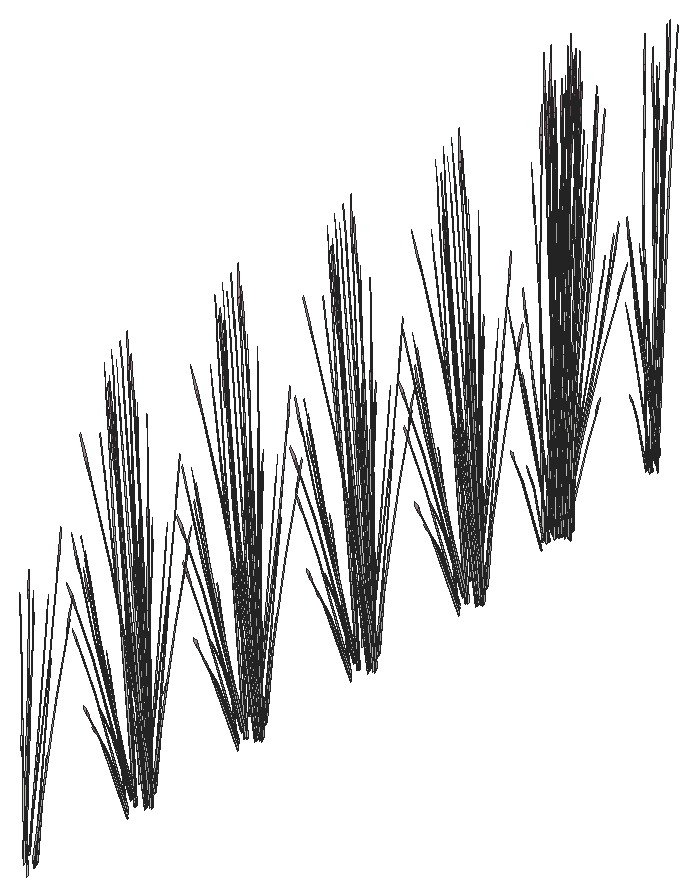
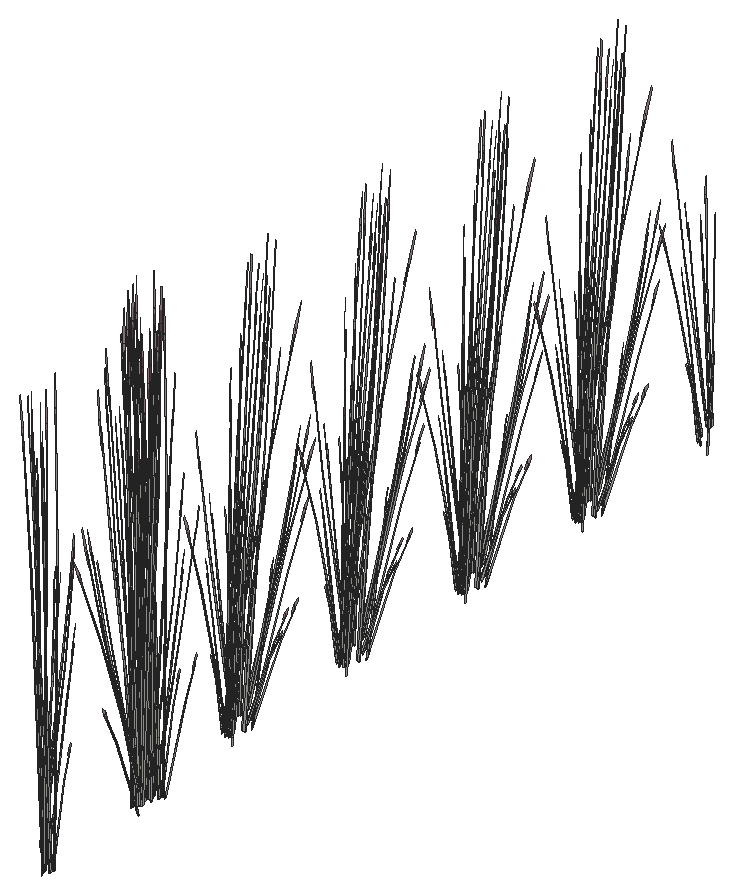
# SketchUp Ruby script. Lengths in inches.
U = 1.inch
M = Sketchup.active_model
def pt(a) = Geom::Point3d.new(a.map { |v| v * U })
def face(e, loops, mat)
  f = e.add_face(loops[0].map { |a| pt(a) })
  loops[1..].each { |l| e.add_face(l.map { |a| pt(a) }).erase! }
  f.material = f.back_material = mat if mat
  f
end
# faces: each face lists its corners as indices into pts; further lists are holes
def faces(e, pts, list, mat = nil) = list.each { |f| face(e, (f[0].is_a?(Array) ? f : [f]).map { |l| l.map { |i| pts[i] } }, mat) }
# xy, xz, yz: faces in a plane at the given z, y or x. An outline is a flat list of corners, or four numbers for a rectangle; further outlines are holes
def ring(l) = l.size == 4 ? [[l[0], l[1]], [l[2], l[1]], [l[2], l[3]], [l[0], l[3]]] : l.each_slice(2).to_a
def flat(e, list, mat, &to3) = list.each { |f| face(e, (f[0].is_a?(Array) ? f : [f]).map { |l| ring(l).map { |u, v| to3.(u, v) } }, mat) }
def xy(e, z, list, mat = nil) = flat(e, list, mat) { |x, y| [x, y, z] }
def xz(e, y, list, mat = nil) = flat(e, list, mat) { |x, z| [x, y, z] }
def yz(e, x, list, mat = nil) = flat(e, list, mat) { |y, z| [x, y, z] }
def lines(e, pts, list) = list.each { |a, b| e.add_line(pt(pts[a]), pt(pts[b])) }
# prism: a flat outline (further loops are holes) pulled along v
def prism(e, loops, v, mat = nil)
  f = face(e, loops, mat); d = Geom::Vector3d.new(v.map { |x| x * U })
  f.pushpull(f.normal.samedirection?(d) ? d.length : -d.length)
end
def box(e, o, s, mat = nil) = prism(e, [[o, [o[0] + s[0], o[1], o[2]], [o[0] + s[0], o[1] + s[1], o[2]], [o[0], o[1] + s[1], o[2]]]], [0, 0, s[2]], mat)
def at(x, y, z, deg = 0) = Geom::Transformation.translation(pt([x, y, z])) * Geom::Transformation.rotation(ORIGIN, Z_AXIS, deg.degrees)
def axes(o, x, y, z) = Geom::Transformation.new([*x, 0, *y, 0, *z, 0, *pt(o).to_a, 1])
def part(name) = M.definitions.add(name)
# library, detail: a bought-in or finely detailed component or shape, given as its bounding box
def library(name, o, s) = part(name).tap { |d| box(d.entities, o, s) }
def detail(e, o, s) = box(e.add_group.entities, o, s)
def put(e, d, t, mat = nil) = e.add_instance(d, t).tap { |i| i.material = mat if mat }
def group(e, t, mat = nil) = e.add_group.tap { |g| g.transformation = t; g.material = mat if mat }.entities
root = M.entities
M.materials.add("LightPink_Translucent").color = [144, 107, 117]
M.materials["LightPink_Translucent"].alpha = 0.75
c1 = part("blade")
p = [[2.15,0.21,22],[0,0.17,0],[0.09,0.45,0],[2.18,0.31,22],[2.29,0.31,22],[0.38,0.45,0],
  [2.48,0.24,33],[2.49,0.24,33],[2.48,0.22,33]]
faces(c1.entities,p,[[0,1,2,3],[4,5,2,3],[6,3,4,7],[8,0,3,6]])
c2 = part("seeds")
p = [[0.3,-0.1,1.38],[-0.01,-0.03,1.59],[-0.01,-0.03,0.03],[0.14,-0.07,-0.07],[0.29,-0.03,3],[0.15,0.01,3.11]]
faces(c2.entities,p,[[0,1,2,3],[1,0,4,5]],"LightPink_Translucent")
c3 = part("blade with seeds")
put(c3.entities,c1,at(0,0,0))
put(c3.entities,c2,axes([2.4,0.25,30.99],[1.5799,-0.05474,1.17369],[-0.12525,1.92788,0.29478],[-0.07173,-0.02425,1.56792]))
put(root,c3,axes([400.97,80.07,3.875],[0.08815,-0.14329,1.71376],[0.22258,0.38678,0.13857],[-0.15267,0.17614,0.73262]))
put(root,c3,axes([400.6875,80.49,4.68],[0.09067,0.42583,-0.51099],[-0.34336,0.07449,-0.3958],[-0.0984,0.11438,0.97773]))
put(root,c3,axes([400.27,81.58,1.49],[0.04734,0.04659,1.76342],[0.08027,0.4317,-0.26939],[-0.10492,0.09206,0.30037]))
put(root,c3,axes([400.9,80.42,3.875],[0.06572,-0.16029,1.71376],[0.27569,0.33172,0.13857],[-0.12437,0.20675,0.73262]))
put(root,c3,axes([400.98,81.33,4.53],[-0.23881,0.24554,-0.35414],[-0.22606,-0.28036,0.4572],[-0.0344,0.14245,0.87481]))
put(root,c3,axes([401.13,82.28,2.77],[-0.00913,-0.2773,1.1486],[0.22824,0.19778,0.84392],[-0.04489,0.13217,0.25299]))
put(root,c3,axes([401.13,81.07,5.34],[-0.00918,0.43138,-0.7886],[-0.38672,-0.02897,0.09517],[-0.04081,0.18275,1.11556]))
put(root,c3,axes([400.86,82.03,2.59],[0.11138,-0.07357,1.43002],[0.27499,0.22183,-0.30754],[-0.08185,0.19194,0.61141]))
put(root,c3,axes([401.01,81.67,3.36],[0.00775,-0.24075,1.54345],[0.34877,0.12716,0.21329],[-0.03022,0.25658,0.72882]))
put(root,c3,axes([401.27,99.36,3.875],[0.08068,0.14973,1.71376],[-0.3728,0.12606,0.13857],[-0.08426,-0.23506,0.73262]))
put(root,c3,axes([401.17,98.96,2.59],[-0.02137,0.15256,1.43002],[-0.31245,0.12771,-0.30754],[-0.07303,-0.19719,0.61141]))
put(root,c3,axes([401.0625,98.72,2.77],[0.18411,0.16231,1.1486],[-0.26813,0.09757,0.84392],[-0.05737,-0.12474,0.25299]))
put(root,c3,axes([401.51,99.58,4.98],[-0.30095,-0.22541,-0.71045],[0.21388,-0.395,0.08574],[-0.10904,-0.13459,1.00501]))
put(root,c3,axes([401.4,99.28,4.53],[-0.05451,-0.37564,-0.35414],[0.31161,-0.09919,0.4572],[-0.0837,-0.10765,0.87481]))
put(root,c3,axes([400.92,99.21,1.49],[-0.03419,0.06144,1.76342],[-0.3455,0.13246,-0.26939],[-0.08346,-0.12049,0.30037]))
put(root,c3,axes([401.37,99.59,4.68],[-0.34827,0.11086,-0.51099],[-0.06092,-0.41983,-0.3958],[-0.09354,-0.12031,0.97773]))
put(root,c3,axes([402.23,102.13,3.33],[0.305,0.18805,1.51261],[-0.29879,0.40513,0.59816],[-0.13384,-0.24012,1.26806]))
put(root,c3,axes([400.68,99.94,4.53],[-0.20082,-0.29199,-0.35414],[0.2293,-0.2764,0.4572],[-0.1165,-0.04206,0.87481]))
put(root,c3,axes([400.7,99.44,2.13],[-0.10181,0.3808,-0.03893],[-0.31336,-0.11714,-0.17649],[-0.04758,-0.06228,0.58215]))
put(root,c3,axes([400.53,101.18,2.375],[-0.44133,0,0],[0,-0.52122,-0.51607],[0,-0.11871,1.63711]))
put(root,c3,axes([400.875,101.04,2.33],[-0.32829,0.39208,0.30756],[-0.32849,-0.38796,-0.36492],[-0.01146,-0.11134,1.64885]))
put(root,c3,axes([401.77,101.86,2.4375],[0.09355,-0.55261,-0.23429],[0.44354,0.09633,0.51271],[-0.0775,-0.07631,1.5644]))
put(root,c3,axes([400.2,100.64,2.77],[0.22533,-0.03337,1.1486],[-0.14293,0.29403,0.84392],[-0.11135,-0.04411,0.25299]))
put(root,c3,axes([401.73,101.64,2.21],[-0.21202,-0.39143,-0.44739],[0.32115,-0.27564,0.21531],[-0.06861,-0.04843,1.43643]))
put(root,c3,axes([401.54,101.79,2.06],[-0.36714,-0.07646,-0.62353],[0.07747,-0.47163,-0.16365],[-0.10956,-0.05715,1.37633]))
put(root,c3,axes([401.15,102.51,2.03],[-0.08291,-0.40636,-0.30978],[0.32928,-0.11539,0.30978],[-0.06638,-0.04686,1.38974]))
put(root,c3,axes([401.0625,102.68,2.02],[-0.33032,-0.23318,-0.49651],[0.19744,-0.41812,0],[-0.07523,-0.05311,1.57504]))
put(root,c3,axes([401.96,101.86,2.67],[-0.35635,0.30962,-0.29095],[-0.23697,-0.43749,-0.50002],[-0.08792,-0.04443,1.59708]))
put(root,c3,axes([402.36,102,2.46],[-0.34464,-0.37536,-0.25192],[0.29,-0.42149,0.5513],[-0.0928,0.04391,1.68216]))
put(root,c3,axes([401.45,102.72,2.48],[0.33032,0.23318,0.49651],[-0.19744,0.41812,0],[-0.07523,-0.05311,1.57504]))
put(root,c3,axes([401.26,102.96,2.375],[-0.22066,0.46731,0],[-0.36918,-0.26061,-0.51607],[-0.08408,-0.05936,1.63711]))
put(root,c3,axes([402.1875,101.92,2.21],[-0.38326,0.02879,-0.44739],[-0.03466,-0.47788,0.21531],[-0.06861,0.04843,1.43643]))
put(root,c3,axes([400.43,102.05,4.53],[-0.30722,0.06665,-0.35414],[-0.08112,-0.381,0.4572],[-0.08804,0.10234,0.87481]))
put(root,c3,axes([402.2,102.2,2.06],[-0.23773,0.35053,-0.62353],[-0.29532,-0.31785,-0.16365],[-0.09526,0.08744,1.37633]))
put(root,c3,axes([400.97,101.67,3.875],[0.08815,-0.14329,1.71376],[0.22258,0.38678,0.13857],[-0.15267,0.17614,0.73262]))
put(root,c3,axes([400.6875,102.09,4.68],[0.09067,0.42583,-0.51099],[-0.34336,0.07449,-0.3958],[-0.0984,0.11438,0.97773]))
put(root,c3,axes([400.27,103.18,1.49],[0.04734,0.04659,1.76342],[0.08027,0.4317,-0.26939],[-0.10492,0.09206,0.30037]))
put(root,c3,axes([400.9,102.03,3.875],[0.06572,-0.16029,1.71376],[0.27569,0.33172,0.13857],[-0.12437,0.20675,0.73262]))
put(root,c3,axes([400.98,102.93,4.53],[-0.23881,0.24554,-0.35414],[-0.22606,-0.28036,0.4572],[-0.0344,0.14245,0.87481]))
put(root,c3,axes([401.13,103.88,2.77],[-0.00913,-0.2773,1.1486],[0.22824,0.19778,0.84392],[-0.04489,0.13217,0.25299]))
put(root,c3,axes([401.13,102.67,5.34],[-0.00918,0.43138,-0.7886],[-0.38672,-0.02897,0.09517],[-0.04081,0.18275,1.11556]))
put(root,c3,axes([400.86,103.64,2.59],[0.11138,-0.07357,1.43002],[0.27499,0.22183,-0.30754],[-0.08185,0.19194,0.61141]))
put(root,c3,axes([401.01,103.28,3.36],[0.00775,-0.24075,1.54345],[0.34877,0.12716,0.21329],[-0.03022,0.25658,0.72882]))
put(root,c3,axes([401.27,119.45,3.875],[0.08068,0.14973,1.71376],[-0.3728,0.12606,0.13857],[-0.08426,-0.23506,0.73262]))
put(root,c3,axes([401.17,119.06,2.59],[-0.02137,0.15256,1.43002],[-0.31245,0.12771,-0.30754],[-0.07303,-0.19719,0.61141]))
put(root,c3,axes([401.0625,118.81,2.77],[0.18411,0.16231,1.1486],[-0.26813,0.09757,0.84392],[-0.05737,-0.12474,0.25299]))
put(root,c3,axes([401.51,119.67,4.98],[-0.30095,-0.22541,-0.71045],[0.21388,-0.395,0.08574],[-0.10904,-0.13459,1.00501]))
put(root,c3,axes([401.4,119.37,4.53],[-0.05451,-0.37564,-0.35414],[0.31161,-0.09919,0.4572],[-0.0837,-0.10765,0.87481]))
put(root,c3,axes([400.92,119.3,1.49],[-0.03419,0.06144,1.76342],[-0.3455,0.13246,-0.26939],[-0.08346,-0.12049,0.30037]))
put(root,c3,axes([401.37,119.68,4.68],[-0.34827,0.11086,-0.51099],[-0.06092,-0.41983,-0.3958],[-0.09354,-0.12031,0.97773]))
put(root,c3,axes([402.23,122.22,3.33],[0.305,0.18805,1.51261],[-0.29879,0.40513,0.59816],[-0.13384,-0.24012,1.26806]))
put(root,c3,axes([400.68,120.03,4.53],[-0.20082,-0.29199,-0.35414],[0.2293,-0.2764,0.4572],[-0.1165,-0.04206,0.87481]))
put(root,c3,axes([400.7,119.54,2.13],[-0.10181,0.3808,-0.03893],[-0.31336,-0.11714,-0.17649],[-0.04758,-0.06228,0.58215]))
put(root,c3,axes([400.53,121.27,2.375],[-0.44133,0,0],[0,-0.52122,-0.51607],[0,-0.11871,1.63711]))
put(root,c3,axes([400.875,121.14,2.33],[-0.32829,0.39208,0.30756],[-0.32849,-0.38796,-0.36492],[-0.01146,-0.11134,1.64885]))
put(root,c3,axes([401.77,121.95,2.4375],[0.09355,-0.55261,-0.23429],[0.44354,0.09633,0.51271],[-0.0775,-0.07631,1.5644]))
put(root,c3,axes([400.2,120.73,2.77],[0.22533,-0.03337,1.1486],[-0.14293,0.29403,0.84392],[-0.11135,-0.04411,0.25299]))
put(root,c3,axes([401.73,121.73,2.21],[-0.21202,-0.39143,-0.44739],[0.32115,-0.27564,0.21531],[-0.06861,-0.04843,1.43643]))
put(root,c3,axes([401.54,121.88,2.06],[-0.36714,-0.07646,-0.62353],[0.07747,-0.47163,-0.16365],[-0.10956,-0.05715,1.37633]))
put(root,c3,axes([401.15,122.6,2.03],[-0.08291,-0.40636,-0.30978],[0.32928,-0.11539,0.30978],[-0.06638,-0.04686,1.38974]))
put(root,c3,axes([401.0625,122.77,2.02],[-0.33032,-0.23318,-0.49651],[0.19744,-0.41812,0],[-0.07523,-0.05311,1.57504]))
put(root,c3,axes([401.96,121.95,2.67],[-0.35635,0.30962,-0.29095],[-0.23697,-0.43749,-0.50002],[-0.08792,-0.04443,1.59708]))
put(root,c3,axes([402.36,122.09,2.46],[-0.34464,-0.37536,-0.25192],[0.29,-0.42149,0.5513],[-0.0928,0.04391,1.68216]))
put(root,c3,axes([401.45,122.81,2.48],[0.33032,0.23318,0.49651],[-0.19744,0.41812,0],[-0.07523,-0.05311,1.57504]))
put(root,c3,axes([401.26,123.05,2.375],[-0.22066,0.46731,0],[-0.36918,-0.26061,-0.51607],[-0.08408,-0.05936,1.63711]))
put(root,c3,axes([402.1875,122.01,2.21],[-0.38326,0.02879,-0.44739],[-0.03466,-0.47788,0.21531],[-0.06861,0.04843,1.43643]))
put(root,c3,axes([400.43,122.14,4.53],[-0.30722,0.06665,-0.35414],[-0.08112,-0.381,0.4572],[-0.08804,0.10234,0.87481]))
put(root,c3,axes([402.2,122.29,2.06],[-0.23773,0.35053,-0.62353],[-0.29532,-0.31785,-0.16365],[-0.09526,0.08744,1.37633]))
put(root,c3,axes([400.97,121.77,3.875],[0.08815,-0.14329,1.71376],[0.22258,0.38678,0.13857],[-0.15267,0.17614,0.73262]))
put(root,c3,axes([400.6875,122.19,4.68],[0.09067,0.42583,-0.51099],[-0.34336,0.07449,-0.3958],[-0.0984,0.11438,0.97773]))
put(root,c3,axes([400.27,123.27,1.49],[0.04734,0.04659,1.76342],[0.08027,0.4317,-0.26939],[-0.10492,0.09206,0.30037]))
put(root,c3,axes([400.9,122.12,3.875],[0.06572,-0.16029,1.71376],[0.27569,0.33172,0.13857],[-0.12437,0.20675,0.73262]))
put(root,c3,axes([400.98,123.02,4.53],[-0.23881,0.24554,-0.35414],[-0.22606,-0.28036,0.4572],[-0.0344,0.14245,0.87481]))
put(root,c3,axes([401.13,123.98,2.77],[-0.00913,-0.2773,1.1486],[0.22824,0.19778,0.84392],[-0.04489,0.13217,0.25299]))
put(root,c3,axes([401.13,122.76,5.34],[-0.00918,0.43138,-0.7886],[-0.38672,-0.02897,0.09517],[-0.04081,0.18275,1.11556]))
put(root,c3,axes([400.86,123.73,2.59],[0.11138,-0.07357,1.43002],[0.27499,0.22183,-0.30754],[-0.08185,0.19194,0.61141]))
put(root,c3,axes([401.01,123.37,3.36],[0.00775,-0.24075,1.54345],[0.34877,0.12716,0.21329],[-0.03022,0.25658,0.72882]))
put(root,c3,axes([401.27,139.9,3.875],[0.08068,0.14973,1.71376],[-0.3728,0.12606,0.13857],[-0.08426,-0.23506,0.73262]))
put(root,c3,axes([401.17,139.5,2.59],[-0.02137,0.15256,1.43002],[-0.31245,0.12771,-0.30754],[-0.07303,-0.19719,0.61141]))
put(root,c3,axes([401.0625,139.26,2.77],[0.18411,0.16231,1.1486],[-0.26813,0.09757,0.84392],[-0.05737,-0.12474,0.25299]))
put(root,c3,axes([401.51,140.12,4.98],[-0.30095,-0.22541,-0.71045],[0.21388,-0.395,0.08574],[-0.10904,-0.13459,1.00501]))
put(root,c3,axes([401.4,139.82,4.53],[-0.05451,-0.37564,-0.35414],[0.31161,-0.09919,0.4572],[-0.0837,-0.10765,0.87481]))
put(root,c3,axes([400.92,139.75,1.49],[-0.03419,0.06144,1.76342],[-0.3455,0.13246,-0.26939],[-0.08346,-0.12049,0.30037]))
put(root,c3,axes([401.37,140.13,4.68],[-0.34827,0.11086,-0.51099],[-0.06092,-0.41983,-0.3958],[-0.09354,-0.12031,0.97773]))
put(root,c3,axes([402.23,142.67,3.33],[0.305,0.18805,1.51261],[-0.29879,0.40513,0.59816],[-0.13384,-0.24012,1.26806]))
put(root,c3,axes([400.68,140.48,4.53],[-0.20082,-0.29199,-0.35414],[0.2293,-0.2764,0.4572],[-0.1165,-0.04206,0.87481]))
put(root,c3,axes([400.7,139.98,2.13],[-0.10181,0.3808,-0.03893],[-0.31336,-0.11714,-0.17649],[-0.04758,-0.06228,0.58215]))
put(root,c3,axes([400.53,141.72,2.375],[-0.44133,0,0],[0,-0.52122,-0.51607],[0,-0.11871,1.63711]))
put(root,c3,axes([400.875,141.59,2.33],[-0.32829,0.39208,0.30756],[-0.32849,-0.38796,-0.36492],[-0.01146,-0.11134,1.64885]))
put(root,c3,axes([401.77,142.4,2.4375],[0.09355,-0.55261,-0.23429],[0.44354,0.09633,0.51271],[-0.0775,-0.07631,1.5644]))
put(root,c3,axes([400.2,141.18,2.77],[0.22533,-0.03337,1.1486],[-0.14293,0.29403,0.84392],[-0.11135,-0.04411,0.25299]))
put(root,c3,axes([401.73,142.18,2.21],[-0.21202,-0.39143,-0.44739],[0.32115,-0.27564,0.21531],[-0.06861,-0.04843,1.43643]))
put(root,c3,axes([401.54,142.33,2.06],[-0.36714,-0.07646,-0.62353],[0.07747,-0.47163,-0.16365],[-0.10956,-0.05715,1.37633]))
put(root,c3,axes([401.15,143.05,2.03],[-0.08291,-0.40636,-0.30978],[0.32928,-0.11539,0.30978],[-0.06638,-0.04686,1.38974]))
put(root,c3,axes([401.0625,143.22,2.02],[-0.33032,-0.23318,-0.49651],[0.19744,-0.41812,0],[-0.07523,-0.05311,1.57504]))
put(root,c3,axes([401.96,142.4,2.67],[-0.35635,0.30962,-0.29095],[-0.23697,-0.43749,-0.50002],[-0.08792,-0.04443,1.59708]))
put(root,c3,axes([402.36,142.54,2.46],[-0.34464,-0.37536,-0.25192],[0.29,-0.42149,0.5513],[-0.0928,0.04391,1.68216]))
put(root,c3,axes([401.45,143.26,2.48],[0.33032,0.23318,0.49651],[-0.19744,0.41812,0],[-0.07523,-0.05311,1.57504]))
put(root,c3,axes([401.26,143.5,2.375],[-0.22066,0.46731,0],[-0.36918,-0.26061,-0.51607],[-0.08408,-0.05936,1.63711]))
put(root,c3,axes([402.1875,142.46,2.21],[-0.38326,0.02879,-0.44739],[-0.03466,-0.47788,0.21531],[-0.06861,0.04843,1.43643]))
put(root,c3,axes([400.43,142.59,4.53],[-0.30722,0.06665,-0.35414],[-0.08112,-0.381,0.4572],[-0.08804,0.10234,0.87481]))
put(root,c3,axes([402.2,142.74,2.06],[-0.23773,0.35053,-0.62353],[-0.29532,-0.31785,-0.16365],[-0.09526,0.08744,1.37633]))
put(root,c3,axes([400.97,142.21,3.875],[0.08815,-0.14329,1.71376],[0.22258,0.38678,0.13857],[-0.15267,0.17614,0.73262]))
put(root,c3,axes([400.6875,142.63,4.68],[0.09067,0.42583,-0.51099],[-0.34336,0.07449,-0.3958],[-0.0984,0.11438,0.97773]))
put(root,c3,axes([400.27,143.72,1.49],[0.04734,0.04659,1.76342],[0.08027,0.4317,-0.26939],[-0.10492,0.09206,0.30037]))
put(root,c3,axes([400.9,142.57,3.875],[0.06572,-0.16029,1.71376],[0.27569,0.33172,0.13857],[-0.12437,0.20675,0.73262]))
put(root,c3,axes([400.98,143.47,4.53],[-0.23881,0.24554,-0.35414],[-0.22606,-0.28036,0.4572],[-0.0344,0.14245,0.87481]))
put(root,c3,axes([401.13,144.43,2.77],[-0.00913,-0.2773,1.1486],[0.22824,0.19778,0.84392],[-0.04489,0.13217,0.25299]))
put(root,c3,axes([401.13,143.21,5.34],[-0.00918,0.43138,-0.7886],[-0.38672,-0.02897,0.09517],[-0.04081,0.18275,1.11556]))
put(root,c3,axes([400.86,144.18,2.59],[0.11138,-0.07357,1.43002],[0.27499,0.22183,-0.30754],[-0.08185,0.19194,0.61141]))
put(root,c3,axes([401.01,143.82,3.36],[0.00775,-0.24075,1.54345],[0.34877,0.12716,0.21329],[-0.03022,0.25658,0.72882]))
put(root,c3,axes([401.27,159.59,3.875],[0.08068,0.14973,1.71376],[-0.3728,0.12606,0.13857],[-0.08426,-0.23506,0.73262]))
put(root,c3,axes([401.17,159.2,2.59],[-0.02137,0.15256,1.43002],[-0.31245,0.12771,-0.30754],[-0.07303,-0.19719,0.61141]))
put(root,c3,axes([401.0625,158.95,2.77],[0.18411,0.16231,1.1486],[-0.26813,0.09757,0.84392],[-0.05737,-0.12474,0.25299]))
put(root,c3,axes([401.51,159.8125,4.98],[-0.30095,-0.22541,-0.71045],[0.21388,-0.395,0.08574],[-0.10904,-0.13459,1.00501]))
put(root,c3,axes([401.4,159.51,4.53],[-0.05451,-0.37564,-0.35414],[0.31161,-0.09919,0.4572],[-0.0837,-0.10765,0.87481]))
put(root,c3,axes([400.92,159.44,1.49],[-0.03419,0.06144,1.76342],[-0.3455,0.13246,-0.26939],[-0.08346,-0.12049,0.30037]))
put(root,c3,axes([401.37,159.82,4.68],[-0.34827,0.11086,-0.51099],[-0.06092,-0.41983,-0.3958],[-0.09354,-0.12031,0.97773]))
put(root,c3,axes([402.23,162.36,3.33],[0.305,0.18805,1.51261],[-0.29879,0.40513,0.59816],[-0.13384,-0.24012,1.26806]))
put(root,c3,axes([400.68,160.18,4.53],[-0.20082,-0.29199,-0.35414],[0.2293,-0.2764,0.4572],[-0.1165,-0.04206,0.87481]))
put(root,c3,axes([400.7,159.68,2.13],[-0.10181,0.3808,-0.03893],[-0.31336,-0.11714,-0.17649],[-0.04758,-0.06228,0.58215]))
put(root,c3,axes([400.53,161.42,2.375],[-0.44133,0,0],[0,-0.52122,-0.51607],[0,-0.11871,1.63711]))
put(root,c3,axes([400.875,161.28,2.33],[-0.32829,0.39208,0.30756],[-0.32849,-0.38796,-0.36492],[-0.01146,-0.11134,1.64885]))
put(root,c3,axes([400.2,160.875,2.77],[0.22533,-0.03337,1.1486],[-0.14293,0.29403,0.84392],[-0.11135,-0.04411,0.25299]))
put(root,c3,axes([401.73,161.87,2.21],[-0.21202,-0.39143,-0.44739],[0.32115,-0.27564,0.21531],[-0.06861,-0.04843,1.43643]))
put(root,c3,axes([401.54,162.02,2.06],[-0.36714,-0.07646,-0.62353],[0.07747,-0.47163,-0.16365],[-0.10956,-0.05715,1.37633]))
put(root,c3,axes([401.15,162.74,2.03],[-0.08291,-0.40636,-0.30978],[0.32928,-0.11539,0.30978],[-0.06638,-0.04686,1.38974]))
put(root,c3,axes([401.0625,162.92,2.02],[-0.33032,-0.23318,-0.49651],[0.19744,-0.41812,0],[-0.07523,-0.05311,1.57504]))
put(root,c3,axes([401.96,162.09,2.67],[-0.35635,0.30962,-0.29095],[-0.23697,-0.43749,-0.50002],[-0.08792,-0.04443,1.59708]))
put(root,c3,axes([402.36,162.23,2.46],[-0.34464,-0.37536,-0.25192],[0.29,-0.42149,0.5513],[-0.0928,0.04391,1.68216]))
put(root,c3,axes([401.45,162.95,2.48],[0.33032,0.23318,0.49651],[-0.19744,0.41812,0],[-0.07523,-0.05311,1.57504]))
put(root,c3,axes([401.26,163.2,2.375],[-0.22066,0.46731,0],[-0.36918,-0.26061,-0.51607],[-0.08408,-0.05936,1.63711]))
put(root,c3,axes([402.1875,162.15,2.21],[-0.38326,0.02879,-0.44739],[-0.03466,-0.47788,0.21531],[-0.06861,0.04843,1.43643]))
put(root,c3,axes([400.43,162.28,4.53],[-0.30722,0.06665,-0.35414],[-0.08112,-0.381,0.4572],[-0.08804,0.10234,0.87481]))
put(root,c3,axes([402.2,162.43,2.06],[-0.23773,0.35053,-0.62353],[-0.29532,-0.31785,-0.16365],[-0.09526,0.08744,1.37633]))
put(root,c3,axes([400.97,161.91,3.875],[0.08815,-0.14329,1.71376],[0.22258,0.38678,0.13857],[-0.15267,0.17614,0.73262]))
put(root,c3,axes([400.6875,162.33,4.68],[0.09067,0.42583,-0.51099],[-0.34336,0.07449,-0.3958],[-0.0984,0.11438,0.97773]))
put(root,c3,axes([400.27,163.41,1.49],[0.04734,0.04659,1.76342],[0.08027,0.4317,-0.26939],[-0.10492,0.09206,0.30037]))
put(root,c3,axes([400.9,162.26,3.875],[0.06572,-0.16029,1.71376],[0.27569,0.33172,0.13857],[-0.12437,0.20675,0.73262]))
put(root,c3,axes([400.98,163.17,4.53],[-0.23881,0.24554,-0.35414],[-0.22606,-0.28036,0.4572],[-0.0344,0.14245,0.87481]))
put(root,c3,axes([401.13,164.12,2.77],[-0.00913,-0.2773,1.1486],[0.22824,0.19778,0.84392],[-0.04489,0.13217,0.25299]))
put(root,c3,axes([401.13,162.91,5.34],[-0.00918,0.43138,-0.7886],[-0.38672,-0.02897,0.09517],[-0.04081,0.18275,1.11556]))
put(root,c3,axes([400.86,163.875,2.59],[0.11138,-0.07357,1.43002],[0.27499,0.22183,-0.30754],[-0.08185,0.19194,0.61141]))
put(root,c3,axes([401.01,163.51,3.36],[0.00775,-0.24075,1.54345],[0.34877,0.12716,0.21329],[-0.03022,0.25658,0.72882]))
put(root,c3,axes([399.53,177.64,2.59],[-0.10032,0.0944,1.43002],[-0.30046,-0.16522,-0.30754],[0.05569,-0.20547,0.61141]))
put(root,c3,axes([398.78,177.12,1.49],[-0.0592,0.0168,1.76342],[-0.32738,-0.18913,-0.26939],[0.00549,-0.15776,0.30037]))
put(root,c3,axes([399.1,177.64,4.53],[0.1064,-0.35863,-0.35414],[0.31043,0.1046,0.4572],[-0.02846,-0.14439,0.87481]))
put(root,c3,axes([399.16,176.88,2.77],[0.04528,0.27194,1.1486],[-0.25117,-0.15062,0.84392],[0.02703,-0.13924,0.25299]))
put(root,c3,axes([399.69,178.19,4.68],[-0.25266,-0.31335,-0.51099],[0.2669,-0.27442,-0.3958],[0.03844,-0.15921,0.97773]))
put(root,c3,axes([398.23,178.01,2.375],[-0.22066,-0.46731,0],[0.36918,-0.26061,-0.51607],[0.08408,-0.05936,1.63711]))
put(root,c3,axes([398.53,177.94,2.02],[0.33032,-0.23318,-0.49651],[0.19744,0.41812,0],[0.07523,-0.05311,1.57504]))
put(root,c3,axes([398.51,179.51,2.21],[0.17124,-0.42022,-0.44739],[0.35581,0.20224,0.21531],[0,-0.09687,1.43643]))
put(root,c3,axes([398.67,179.3,2.67],[-0.04113,-0.53214,-0.29095],[0.42835,-0.03218,-0.50002],[0.07543,-0.07088,1.59708]))
put(root,c3,axes([398.61,178.125,2.03],[0.32928,0.11539,-0.30978],[-0.08291,0.40636,0.30978],[0.06638,-0.04686,1.38974]))
put(root,c3,axes([398.72,179.72,2.43],[0.39767,0.22603,0.24065],[-0.19139,0.46966,0.50002],[0,-0.10827,1.60543]))
put(root,c3,axes([398.6,179.41,2.72],[-0.38326,0.02879,0.44739],[-0.03466,-0.47788,-0.21531],[0.06861,-0.04843,1.43643]))
put(root,c3,axes([398.58,179.58,2.36],[0.15345,0.52148,0.45755],[-0.43845,0.18134,0.17955],[0.00536,-0.09582,1.58856]))
put(root,c3,axes([399.13,179.62,2.21],[0,-0.53961,0],[0.44133,0,0],[0,0,1.79456]))
put(root,c3,axes([398.92,179.28,2.36],[-0.29264,0.42323,0.45755],[-0.34767,-0.3736,0.17955],[0.07055,-0.04224,1.58856]))
put(root,c3,axes([399.24,180.04,2.3],[-0.32829,-0.4014,-0.06131],[0.32849,-0.40164,0],[-0.01146,-0.01402,1.75571]))
put(root,c3,axes([398.42,178.59,2.47],[-0.10196,0.46348,0.17642],[-0.3731,-0.13116,0.35086],[0.06445,-0.00226,1.60407]))
put(root,c3,axes([399.2,179.1,2.62],[0.06809,-0.4162,0.1448],[0.33266,0.07225,-0.41347],[0.06054,0.04274,1.26744]))
put(root,c3,axes([399.05,179.21,2.72],[-0.21202,-0.39143,0.44739],[0.32115,-0.27564,-0.21531],[0.06861,0.04843,1.43643]))
put(root,c3,axes([398.38,180.98,2.47],[0.37926,-0.12378,0.17642],[0.09365,0.46065,0.35086],[-0.03382,-0.06712,1.60407]))
put(root,c3,axes([399.43,179.74,2.21],[0.39487,0,0],[0,0.48281,0],[0,0,1.78407]))
put(root,c3,axes([399.55,178.61,2.47],[-0.37926,0.12378,0.17642],[-0.09365,-0.46065,0.35086],[0.03382,0.06712,1.60407]))
put(root,c3,axes([399.31,179.5,2.38],[-0.44609,-0.09826,0.49198],[0.09078,-0.55493,0.19306],[0.06519,0.05359,1.70813]))
put(root,c3,axes([398.95,180.87,2.2],[-0.11516,-0.40207,0],[0.32884,-0.1408,0],[0,0,1.54371]))
put(root,c3,axes([399.51,181,2.47],[0.10196,-0.46348,0.17642],[0.3731,0.13116,0.35086],[-0.06445,0.00226,1.60407]))
put(root,c3,axes([399.42,179.95,2.21],[0.24637,0.30123,0],[-0.24637,0.30123,0],[0,0,1.69266]))
put(root,c3,axes([400.09,179.82,2.47],[-0.2773,-0.3397,0.17642],[0.27945,-0.32949,0.35086],[-0.03063,0.06937,1.60407]))
put(root,c3,axes([398.87,181.05,2.2],[-0.35581,-0.20937,0],[0.17124,-0.43505,0],[0,0,1.62707]))
put(root,c3,axes([399.42,179.6,2.72],[0.17124,-0.42022,0.44739],[0.35581,0.20224,-0.21531],[0,0.09687,1.43643]))
put(root,c3,axes([399.36,179.84,2.29],[0,0.53934,-0.05637],[-0.44133,0,0],[0,0.01695,1.79368]))
put(root,c3,axes([400.32,179.83,2.48],[0,-0.46636,0.49651],[0.39487,0,0],[0,0.10622,1.57504]))
put(root,c3,axes([399.33,180.18,2.72],[0.38326,-0.02879,0.44739],[0.03466,0.47788,-0.21531],[-0.06861,0.04843,1.43643]))
put(root,c3,axes([399.57,179.69,2.62],[0.32884,-0.136,0.1448],[0.11516,0.38837,-0.41347],[0,0.08547,1.26744]))
put(root,c3,axes([399.27,181.06,2.2],[0.35581,0.20937,0],[-0.17124,0.43505,0],[0,0,1.74954]))
put(root,c3,axes([399.34,180.39,2.62],[0.26075,0.2802,0.1448],[-0.2175,0.31612,-0.41347],[-0.06054,0.04274,1.26744]))
put(root,c3,axes([399.61,181.25,2.48],[0.33032,-0.23318,0.49651],[0.19744,0.41812,0],[-0.07523,0.05311,1.57504]))
put(root,c3,axes([399.14,180.88,2.29],[0.15345,0.53576,-0.06012],[-0.43845,0.18773,0],[0.00536,0.01871,1.72173]))
put(root,c3,axes([400.41,180.18,2.2],[-0.44111,-0.00373,-0.04976],[0,-0.52122,0.49943],[-0.01386,0.11865,1.58352]))
put(root,c3,axes([399.46,179.72,2.67],[0.39748,0.22252,-0.29095],[-0.19139,0.46966,-0.50002],[0.01249,0.11531,1.59708]))
put(root,c3,axes([400.32,180.25,2.03],[-0.24637,0.29097,-0.30978],[-0.24637,-0.29097,0.30978],[0,0.09372,1.38974]))
put(root,c3,axes([399.41,180.07,2.21],[-0.17124,0.42022,-0.44739],[-0.35581,-0.20224,0.21531],[0,0.09687,1.43643]))
put(root,c3,axes([399.42,181.28,2.33],[0.44186,0.15158,0.30756],[-0.11054,0.54181,-0.36492],[-0.07313,0.06781,1.64885]))
put(root,c3,axes([400.49,180.26,2.02],[0,0.46636,-0.49651],[-0.39487,0,0],[0,0.10622,1.57504]))
put(root,c3,axes([399.69,181.57,2.375],[0.22066,0.46731,0],[-0.36918,0.26061,-0.51607],[-0.08408,0.05936,1.63711]))
put(root,c3,axes([399.62,180.2,2.09],[0.12941,0.42699,-0.69212],[-0.37279,0.15378,-0.18165],[0.0143,0.14459,1.52773]))
put(root,c3,axes([398.53,181.72,1.49],[0.05712,-0.02538,1.76342],[0.34359,0.13968,-0.26939],[0.01005,0.15742,0.30037]))
put(root,c3,axes([398.77,181.61,4.68],[0.34695,0.11691,-0.51099],[-0.11892,0.40083,-0.3958],[0.03181,0.16138,0.97773]))
put(root,c3,axes([398.96,180.78,3.875],[-0.08068,-0.14973,1.71376],[0.3728,-0.12606,0.13857],[0.08426,0.23506,0.73262]))
put(root,c3,axes([398.61,181.86,4.53],[-0.1064,0.35863,-0.35414],[-0.31043,-0.1046,0.4572],[0.02846,0.14439,0.87481]))
put(root,c3,axes([398.64,181.54,4.98],[0.16845,0.3792,-0.71045],[-0.34676,0.21133,0.08574],[0.03939,0.18322,1.00501]))
put(root,c3,axes([398.51,197.67,2.59],[-0.10032,0.0944,1.43002],[-0.30046,-0.16522,-0.30754],[0.05569,-0.20547,0.61141]))
put(root,c3,axes([398.76,198.37,4.98],[0.00918,-0.43138,-0.71045],[0.38672,0.02897,0.08574],[0.04081,-0.18275,1.00501]))
put(root,c3,axes([398.32,198.15,3.875],[-0.06572,0.16029,1.71376],[-0.27569,-0.33172,0.13857],[0.12437,-0.20675,0.73262]))
put(root,c3,axes([398.14,196.92,2.77],[0.04528,0.27194,1.1486],[-0.25117,-0.15062,0.84392],[0.02703,-0.13924,0.25299]))
put(root,c3,axes([398.68,198.23,4.68],[-0.25266,-0.31335,-0.51099],[0.2669,-0.27442,-0.3958],[0.03844,-0.15921,0.97773]))
put(root,c3,axes([398.92,198.11,4.53],[0.23881,-0.24554,-0.35414],[0.22606,0.28036,0.4572],[0.0344,-0.14245,0.87481]))
put(root,c3,axes([397.22,198.05,2.375],[-0.22066,-0.46731,0],[0.36918,-0.26061,-0.51607],[0.08408,-0.05936,1.63711]))
put(root,c3,axes([397.52,197.98,2.02],[0.33032,-0.23318,-0.49651],[0.19744,0.41812,0],[0.07523,-0.05311,1.57504]))
put(root,c3,axes([397.91,198.93,2.06],[0.23773,-0.35053,-0.62353],[0.29532,0.31785,-0.16365],[0.09526,-0.08744,1.37633]))
put(root,c3,axes([397.65,199.34,2.67],[-0.04113,-0.53214,-0.29095],[0.42835,-0.03218,-0.50002],[0.07543,-0.07088,1.59708]))
put(root,c3,axes([397.6,198.16,2.03],[0.32928,0.11539,-0.30978],[-0.08291,0.40636,0.30978],[0.06638,-0.04686,1.38974]))
put(root,c3,axes([397.58,199.44,2.72],[-0.38326,0.02879,0.44739],[-0.03466,-0.47788,-0.21531],[0.06861,-0.04843,1.43643]))
put(root,c3,axes([398.65,198.41,2.48],[-0.33032,-0.23318,0.49651],[0.19744,-0.41812,0],[0.07523,0.05311,1.57504]))
put(root,c3,axes([397.91,199.32,2.36],[-0.29264,0.42323,0.45755],[-0.34767,-0.3736,0.17955],[0.07055,-0.04224,1.58856]))
put(root,c3,axes([397.4,198.62,2.47],[-0.10196,0.46348,0.17642],[-0.3731,-0.13116,0.35086],[0.06445,-0.00226,1.60407]))
